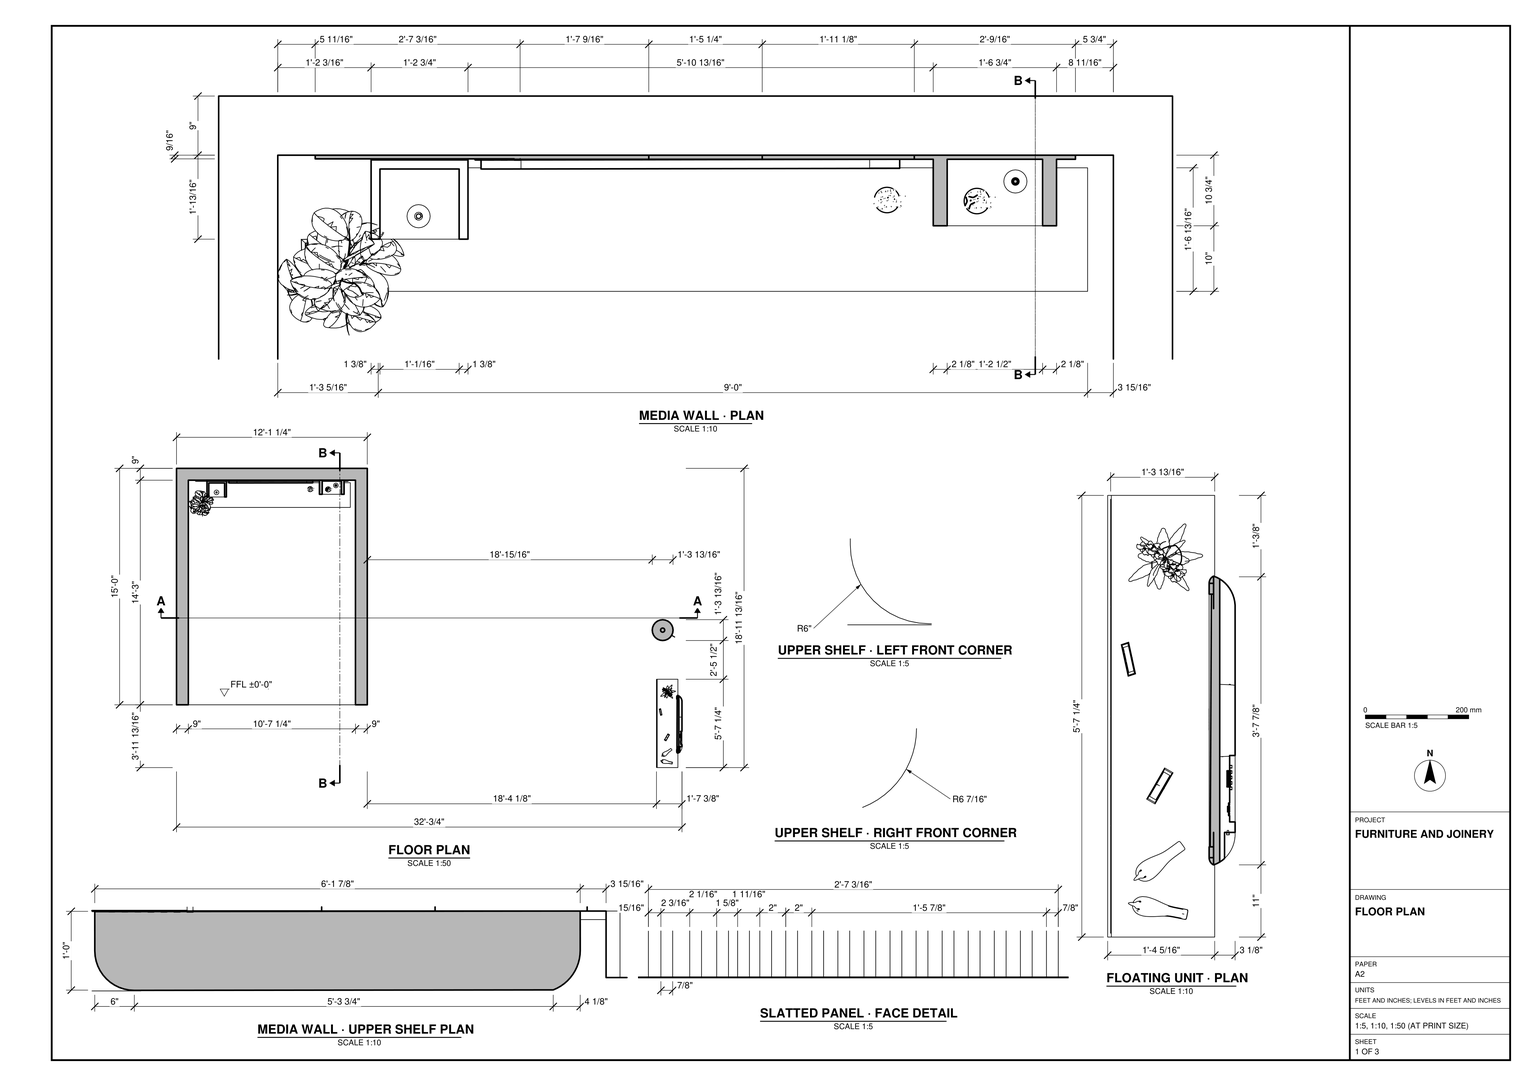
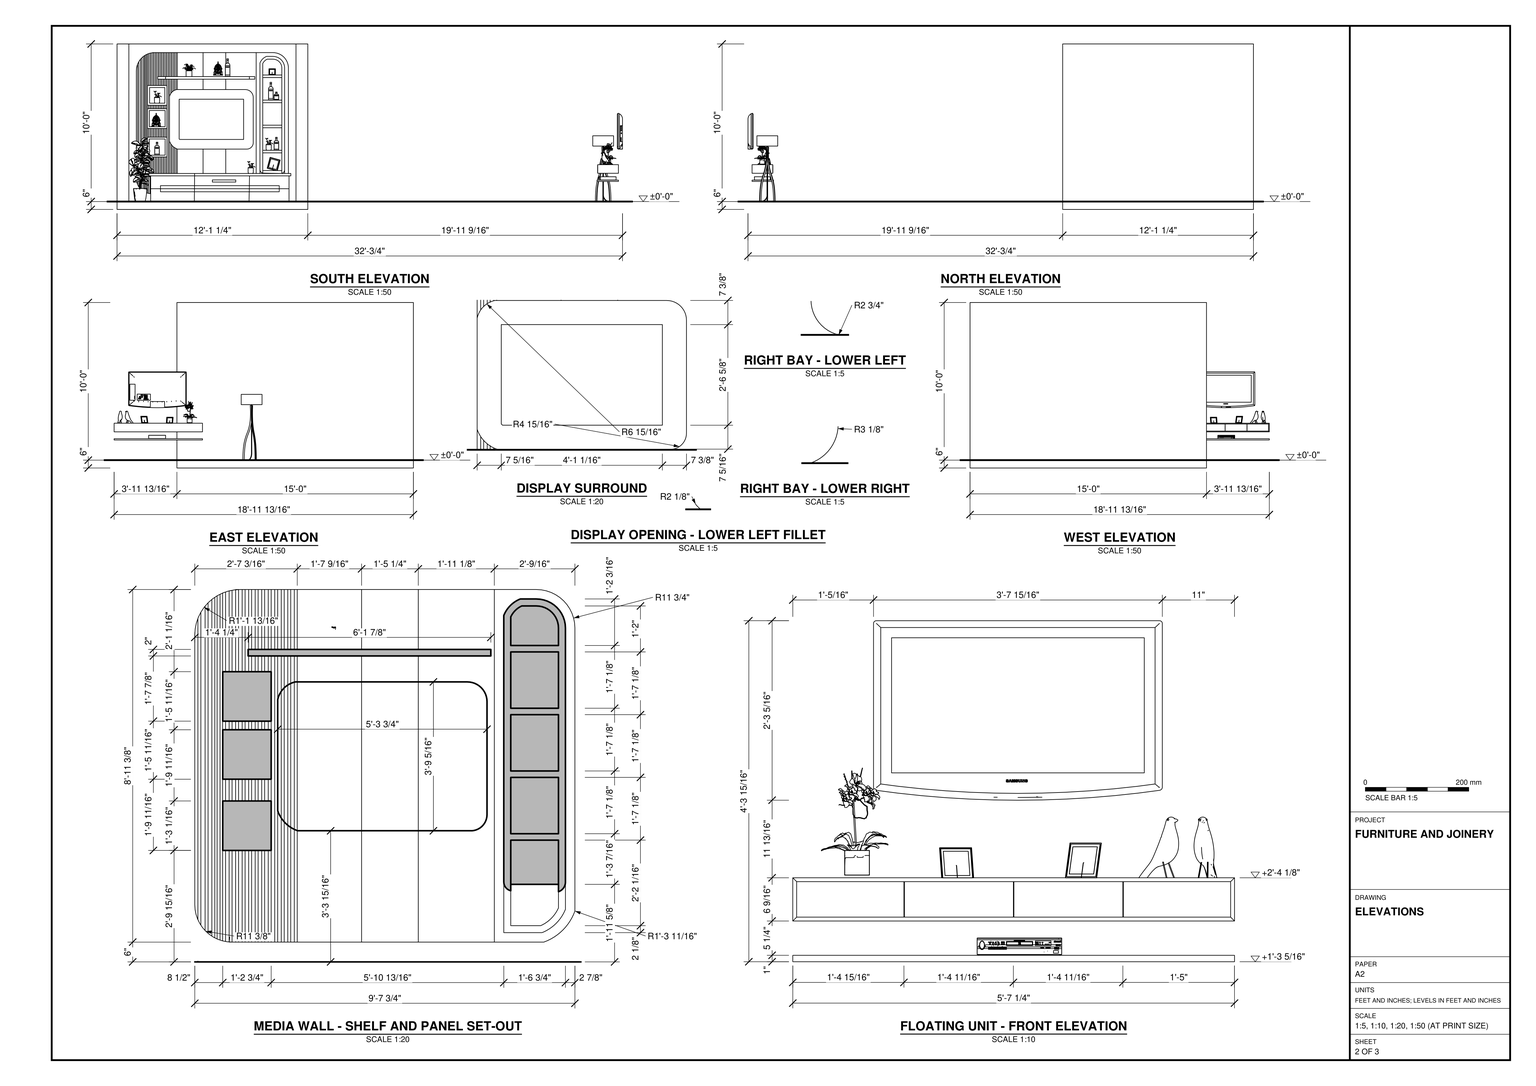
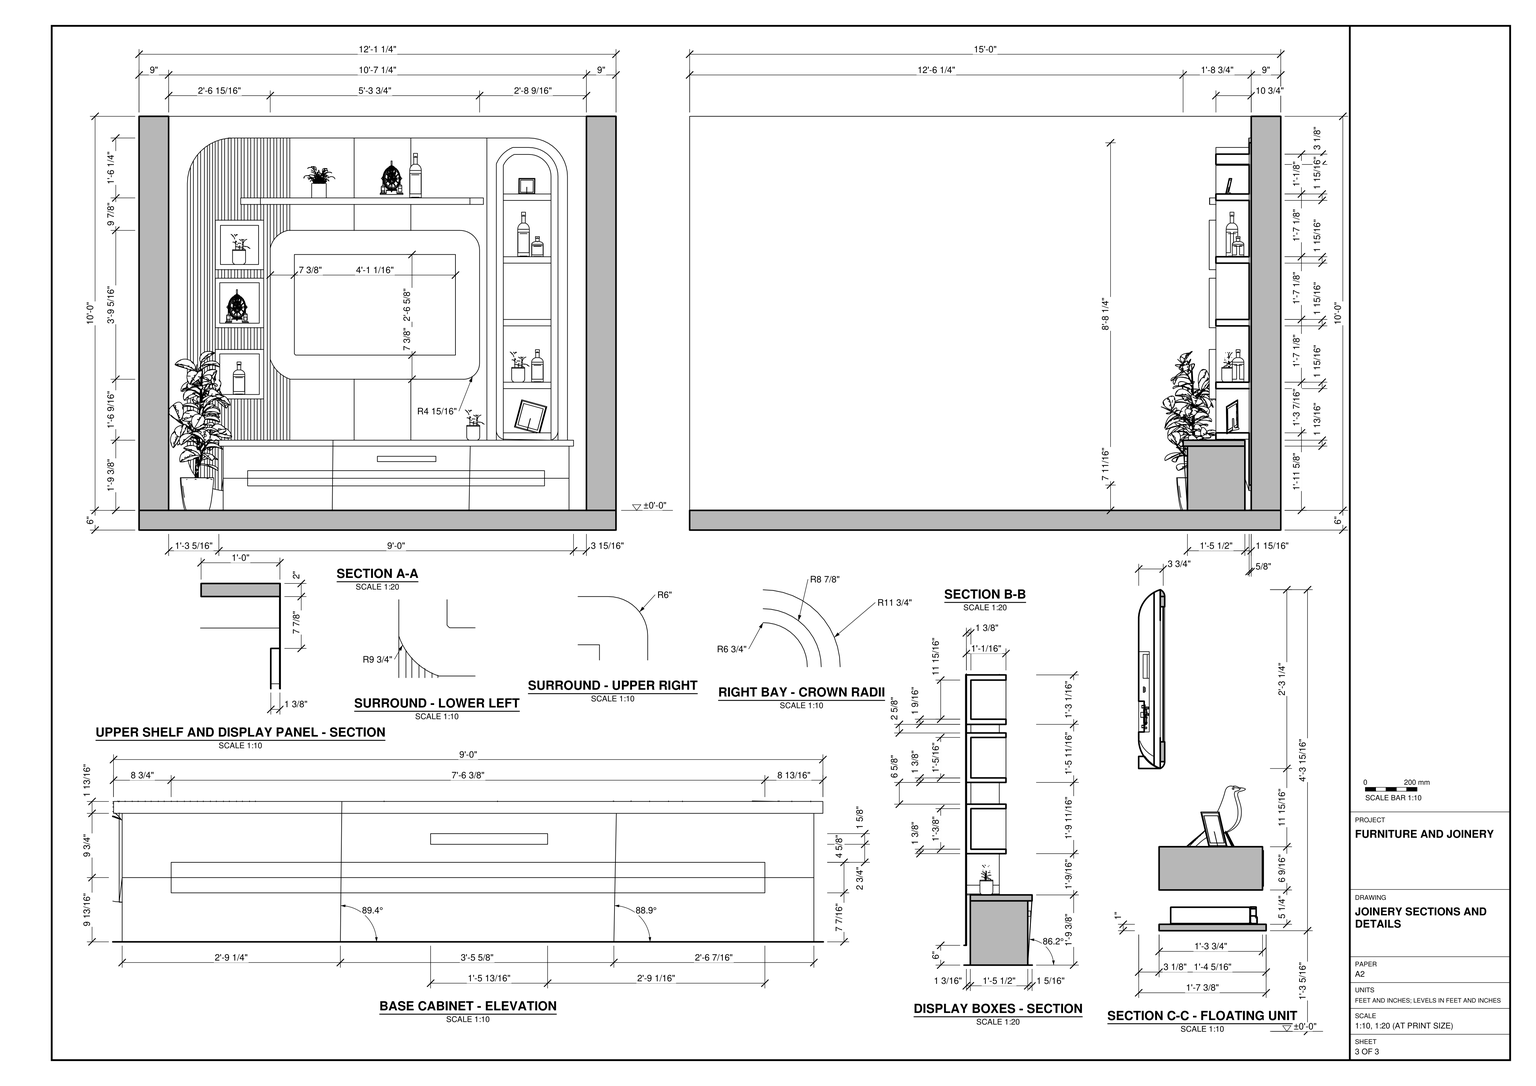
Use task_files/diagram_01.pdf to build the media wall, its enclosure and the separate floating display unit in SketchUp. Work in feet and inches. The complete layout measures 32'-3/4" along x, 18'-11 13/16" along y and 10'-6" in height. Set the single finished floor level at ±0'-0". Model the 6" floor slab and the 9" back and side walls, leaving the front open as shown in plan.

Build the media wall against the back wall. Use the section facing the joinery to align the divided base cabinet, slatted panel, three open display boxes, central display surround and tall right-hand shelving bay. Follow the details for the rounded corners of the surround, the projecting upper shelf and the nested curves at the crown of the shelving bay.

Use the floor plan to position the separate floating unit outside the enclosure, with its length perpendicular to the base cabinet. Include its divided console, lower shelf and display above. Decor and loose items, including plants, clocks, lamps and objects on the shelves, may be any suitable library components placed as shown. Keep the walls, slab and each furniture or joinery piece in separate groups or components, and use components for repeated parts. Save one SketchUp model as output_files/media_wall_and_separate_floating_display_unit.skp.

# SketchUp Ruby script. Lengths in inches.
U = 1.inch
M = Sketchup.active_model
def pt(a) = Geom::Point3d.new(a.map { |v| v * U })
def face(e, loops, mat)
  f = e.add_face(loops[0].map { |a| pt(a) })
  loops[1..].each { |l| e.add_face(l.map { |a| pt(a) }).erase! }
  f.material = f.back_material = mat if mat
  f
end
# faces: each face lists its corners as indices into pts; further lists are holes
def faces(e, pts, list, mat = nil) = list.each { |f| face(e, (f[0].is_a?(Array) ? f : [f]).map { |l| l.map { |i| pts[i] } }, mat) }
# xy, xz, yz: faces in a plane at the given z, y or x. An outline is a flat list of corners, or four numbers for a rectangle; further outlines are holes
def ring(l) = l.size == 4 ? [[l[0], l[1]], [l[2], l[1]], [l[2], l[3]], [l[0], l[3]]] : l.each_slice(2).to_a
def flat(e, list, mat, &to3) = list.each { |f| face(e, (f[0].is_a?(Array) ? f : [f]).map { |l| ring(l).map { |u, v| to3.(u, v) } }, mat) }
def xy(e, z, list, mat = nil) = flat(e, list, mat) { |x, y| [x, y, z] }
def xz(e, y, list, mat = nil) = flat(e, list, mat) { |x, z| [x, y, z] }
def yz(e, x, list, mat = nil) = flat(e, list, mat) { |y, z| [x, y, z] }
def lines(e, pts, list) = list.each { |a, b| e.add_line(pt(pts[a]), pt(pts[b])) }
# prism: a flat outline (further loops are holes) pulled along v
def prism(e, loops, v, mat = nil)
  f = face(e, loops, mat); d = Geom::Vector3d.new(v.map { |x| x * U })
  f.pushpull(f.normal.samedirection?(d) ? d.length : -d.length)
end
def box(e, o, s, mat = nil) = prism(e, [[o, [o[0] + s[0], o[1], o[2]], [o[0] + s[0], o[1] + s[1], o[2]], [o[0], o[1] + s[1], o[2]]]], [0, 0, s[2]], mat)
def at(x, y, z, deg = 0) = Geom::Transformation.translation(pt([x, y, z])) * Geom::Transformation.rotation(ORIGIN, Z_AXIS, deg.degrees)
def axes(o, x, y, z) = Geom::Transformation.new([*x, 0, *y, 0, *z, 0, *pt(o).to_a, 1])
def part(name) = M.definitions.add(name)
# library, detail: a bought-in or finely detailed component or shape, given as its bounding box
def library(name, o, s) = part(name).tap { |d| box(d.entities, o, s) }
def detail(e, o, s) = box(e.add_group.entities, o, s)
def put(e, d, t, mat = nil) = e.add_instance(d, t).tap { |i| i.material = mat if mat }
def group(e, t, mat = nil) = e.add_group.tap { |g| g.transformation = t; g.material = mat if mat }.entities
root = M.entities
M.materials.add("Frame_Pic").color = [0, 0, 0]
M.materials.add("Glossy_White").color = [188, 188, 188]
M.materials.add("Pic_Bed").color = [214, 209, 200]
M.materials.add("White Wall").color = [242, 239, 237]
M.materials.add("White_Fur").color = [226, 226, 226]
M.materials.add("Wood_Fur").color = [191, 176, 157]
M.materials.add("[Blinds Vertical Pattern]").color = [212, 212, 214]
M.materials.add("[Color M00]").color = [255, 255, 255]
M.materials.add("[Color M09]").color = [0, 0, 0]
M.materials.add("[Color_000]1").color = [255, 255, 126]
M.materials.add("[Color_000]2").color = [135, 140, 128]
M.materials.add("[Color_008]1").color = [28, 28, 28]
M.materials.add("[Color_008]2").color = [29, 29, 29]
M.materials.add("[Wood Bamboo]").color = [177, 105, 43]
M.materials.add("kinh1").color = [126, 126, 126]
M.materials["kinh1"].alpha = 0
M.materials.add("model").color = [217, 78, 64]
M.materials.add("product_RG_W___dLorraine_80x80_Kepingan2").color = [228, 228, 223]
c1 = library("Small Plant for Nightstand",[-0.92,-1.74,0],[6.62,5.06,9.81])
c2 = library("PLANT SMALL",[-1.72,-1.35,0],[13.55,13.62,9.59])
c3 = library("SmallMag",[0,-0.13,0],[5.12,2.39,5.75])
c4 = library("Vodka",[0,0,0],[3.53,3.53,13.57])
c5 = library("Group_2",[-1.28,-0.39,0],[21.22,20.51,48.44])
c6 = library("model",[-3.64,-1.86,0],[7.28,3.72,11.8125])
c7 = library("Estante p/ Sala de TV - designed by Tiago Crisostomo",[-3.75,0,10.71],[23.44,133.86,62.71])
c8 = library("Potted orchid",[-4.6,-2.59,0],[19.81,21.87,25.9])
c9 = part("Group\#70")
xy(c9.entities,0,[[0,0,16.59,0.1]],"Glossy_White")
xy(c9.entities,5.4,[[0,0,16.59,0.1]],"Glossy_White")
xz(c9.entities,0,[[0,0,16.59,5.4]])
xz(c9.entities,0.1,[[0,0,16.59,5.4]],"Glossy_White")
yz(c9.entities,0,[[0,0,0.1,5.4]],"Glossy_White")
yz(c9.entities,16.59,[[0,0,0.1,5.4]],"Glossy_White")
c10 = part("Group\#83")
xy(c10.entities,0,[[0.26,0,16.59,0.1]],"Glossy_White")
xy(c10.entities,5.4,[[0.26,0,16.59,0.1]],"Glossy_White")
xz(c10.entities,0,[[0.26,0,16.59,5.4]])
xz(c10.entities,0.1,[[0.26,0,16.59,5.4]],"Glossy_White")
yz(c10.entities,0.26,[[0,0,0.1,5.4]],"Glossy_White")
yz(c10.entities,16.59,[[0,0,0.1,5.4]],"Glossy_White")
c11 = library("Group\#74",[-0.65,-0.12,0],[14.95,9.57,9.38])
c12 = part("Picture frame stand")
prism(c12.entities,[[[0,6.65,1.14],[0,6.68,0.91],[0,6.65,0.68],[0,6.5625,0.47],[0,6.43,0.28],[0,6.25,0.14],[0,6.04,0.04],[0,5.82,0],[0,0,0],[0,2.74,10.21],[0,2.79,10.35],[0,2.87,10.47],[0,2.98,10.57],[0,3.1,10.65],[0,3.24,10.7],[0,3.39,10.71],[0,3.53,10.7],[0,3.67,10.65],[0,3.8,10.57],[0,3.9,10.47],[0,3.99,10.35],[0,4.04,10.21],[0,2.39,3.68],[0,2.35,3.44],[0,2.35,3.2],[0,2.39,2.96],[0,2.47,2.73],[0,2.58,2.51],[0,2.72,2.32],[0,2.9,2.15],[0,3.1,2.01],[0,3.32,1.91],[0,3.55,1.84],[0,3.8,1.81],[0,4.04,1.82],[0,5.82,1.82],[0,6.04,1.78],[0,6.25,1.68],[0,6.43,1.54],[0,6.5625,1.35]]],[0.2,0,0],"Frame_Pic")
c13 = part("Standing picture frame")
yz(c13.entities,0,[[0.38,0,0,0.1,6.52,24.44,6.9,24.34]],"Frame_Pic")
yz(c13.entities,0.79,[[0.58,0.76,6.7,23.58,6.51,23.63,0.39,0.8125],[0.39,0.8125,6.51,23.63,6.32,23.68,0.2,0.86]])
yz(c13.entities,2.76,[[0.9,2.71,0.71,2.76,5.81,21.78,6,21.73]],"[Color_008]1")
yz(c13.entities,22.44,[[0.9,2.71,6,21.73,5.81,21.78,0.71,2.76]],"[Color_008]1")
yz(c13.entities,24.41,[[0.58,0.76,0.39,0.8125,6.51,23.63,6.7,23.58]])
yz(c13.entities,24.41,[[0.39,0.8125,0.2,0.86,6.32,23.68,6.51,23.63]],"[Color_008]1")
yz(c13.entities,25.2,[[0.38,0,6.9,24.34,6.52,24.44,0,0.1]],"Frame_Pic")
p = [[0,0.38,0],[25.2,0.38,0],[25.2,0,0.1],[0,0,0.1],[0,6.9,24.34],[25.2,6.9,24.34],
  [24.41,6.7,23.58],[0.79,6.7,23.58],[0.79,0.58,0.76],[24.41,0.58,0.76],[0,6.52,24.44],[25.2,6.52,24.44],
  [0.79,6.32,23.68],[24.41,6.32,23.68],[24.41,0.2,0.86],[0.79,0.2,0.86],[24.41,0.39,0.8125],[0.79,0.39,0.8125],
  [24.41,6.51,23.63],[0.79,6.51,23.63],[22.44,6,21.73],[22.44,0.9,2.71],[2.76,0.9,2.71],[2.76,6,21.73],
  [2.76,0.71,2.76],[22.44,0.71,2.76],[22.44,5.81,21.78],[2.76,5.81,21.78]]
faces(c13.entities,p,[[0,1,2,3],[[0,4,5,1],[6,7,8,9]],[14,16,17,15],[24,22,21,25],[26,20,23,27]],"[Color_008]1")
faces(c13.entities,p,[[[10,3,2,11],[12,13,14,15]],[5,4,10,11]],"Frame_Pic")
faces(c13.entities,p,[[[16,18,19,17],[20,21,22,23]],[7,6,9,8]],"[Color_000]2")
faces(c13.entities,p,[[9,8,17,16],[21,20,23,22],[12,19,18,13],[7,6,18,19]])
faces(c13.entities,p,[[24,25,26,27]],"Pic_Bed")
put(c13.entities,c12,at(12.6,0.38,0))
c14 = part("Picture frame stand \#1")
prism(c14.entities,[[[0.2,0,0],[0.2,5.82,0],[0.2,6.04,0.04],[0.2,6.25,0.14],[0.2,6.43,0.28],[0.2,6.5625,0.47],[0.2,6.65,0.68],[0.2,6.68,0.91],[0.2,6.65,1.14],[0.2,6.5625,1.35],[0.2,6.43,1.54],[0.2,6.25,1.68],[0.2,6.04,1.78],[0.2,5.82,1.82],[0.2,4.04,1.82],[0.2,3.8,1.81],[0.2,3.55,1.84],[0.2,3.32,1.91],[0.2,3.1,2.01],[0.2,2.9,2.15],[0.2,2.72,2.32],[0.2,2.58,2.51],[0.2,2.47,2.73],[0.2,2.39,2.96],[0.2,2.35,3.2],[0.2,2.35,3.44],[0.2,2.39,3.68],[0.2,4.04,10.21],[0.2,3.99,10.35],[0.2,3.9,10.47],[0.2,3.8,10.57],[0.2,3.67,10.65],[0.2,3.53,10.7],[0.2,3.39,10.71],[0.2,3.24,10.7],[0.2,3.1,10.65],[0.2,2.98,10.57],[0.2,2.87,10.47],[0.2,2.79,10.35],[0.2,2.74,10.21]]],[-0.2,0,0],"[Color_008]1")
c15 = part("Standing picture frame \#1")
yz(c15.entities,0,[[0.38,0,0,0.1,6.52,24.44,6.9,24.34]],"[Color_008]2")
yz(c15.entities,0.79,[[0.58,0.76,6.7,23.58,6.51,23.63,0.39,0.8125],[0.39,0.8125,6.51,23.63,6.32,23.68,0.2,0.86]])
yz(c15.entities,2.76,[[0.9,2.71,0.71,2.76,5.81,21.78,6,21.73]],"[Color_008]2")
yz(c15.entities,22.44,[[0.9,2.71,6,21.73,5.81,21.78,0.71,2.76]],"[Color_008]2")
yz(c15.entities,24.41,[[0.58,0.76,0.39,0.8125,6.51,23.63,6.7,23.58]])
yz(c15.entities,24.41,[[0.39,0.8125,0.2,0.86,6.32,23.68,6.51,23.63]],"[Color_008]2")
yz(c15.entities,25.2,[[0.38,0,6.9,24.34,6.52,24.44,0,0.1]],"[Color_008]2")
p = [[0,0.38,0],[25.2,0.38,0],[25.2,0,0.1],[0,0,0.1],[0,6.9,24.34],[25.2,6.9,24.34],
  [24.41,6.7,23.58],[0.79,6.7,23.58],[0.79,0.58,0.76],[24.41,0.58,0.76],[0,6.52,24.44],[0.05,-0.6,0.22],
  [0.05,5.92,24.55],[25.25,-0.6,0.22],[25.2,6.52,24.44],[25.25,5.92,24.55],[0.84,5.72,23.79],[24.46,5.72,23.79],
  [24.46,-0.4,0.98],[0.84,-0.4,0.98],[24.41,0.2,0.86],[24.41,0.39,0.8125],[0.79,0.39,0.8125],[0.79,0.2,0.86],
  [24.41,6.51,23.63],[0.79,6.51,23.63],[22.44,6,21.73],[22.44,0.9,2.71],[2.76,0.9,2.71],[2.76,6,21.73],
  [0.79,6.32,23.68],[24.41,6.32,23.68],[2.76,0.71,2.76],[22.44,0.71,2.76],[22.44,5.81,21.78],[2.76,5.81,21.78]]
faces(c15.entities,p,[[0,1,2,3],[[0,4,5,1],[6,7,8,9]],[10,3,11,12],[3,2,13,11],[2,14,15,13],[[12,11,13,15],[16,17,18,19]],[20,21,22,23],[23,30,16,19],
  [20,23,19,18],[31,20,18,17],[32,28,27,33],[34,26,29,35],[30,31,17,16],[5,4,10,14],[14,10,12,15]],"[Color_008]2")
faces(c15.entities,p,[[[21,24,25,22],[26,27,28,29]],[7,6,9,8]],"[Color_000]1")
faces(c15.entities,p,[[9,8,22,21],[27,26,29,28],[32,33,34,35],[30,25,24,31],[7,6,24,25]])
put(c15.entities,c14,at(12.6,0.38,0))
c16 = part("Standing picture frame \#2")
yz(c16.entities,0,[[0.38,0,0,0.1,6.52,24.44,6.9,24.34]],"[Color_008]2")
yz(c16.entities,0.79,[[0.58,0.76,6.7,23.58,6.51,23.63,0.39,0.8125],[0.39,0.8125,6.51,23.63,6.32,23.68,0.2,0.86]])
yz(c16.entities,2.76,[[0.9,2.71,0.71,2.76,5.81,21.78,6,21.73]],"[Color_008]2")
yz(c16.entities,22.44,[[0.9,2.71,6,21.73,5.81,21.78,0.71,2.76]],"[Color_008]2")
yz(c16.entities,24.41,[[0.58,0.76,0.39,0.8125,6.51,23.63,6.7,23.58]])
yz(c16.entities,24.41,[[0.39,0.8125,0.2,0.86,6.32,23.68,6.51,23.63]],"[Color_008]2")
yz(c16.entities,25.2,[[0.38,0,6.9,24.34,6.52,24.44,0,0.1]],"[Color_008]2")
p = [[0,0.38,0],[25.2,0.38,0],[25.2,0,0.1],[0,0,0.1],[0,6.9,24.34],[25.2,6.9,24.34],
  [24.41,6.7,23.58],[0.79,6.7,23.58],[0.79,0.58,0.76],[24.41,0.58,0.76],[0,6.52,24.44],[0.05,-0.6,0.22],
  [0.05,5.92,24.55],[25.25,-0.6,0.22],[25.2,6.52,24.44],[25.25,5.92,24.55],[0.84,5.72,23.79],[24.46,5.72,23.79],
  [24.46,-0.4,0.98],[0.84,-0.4,0.98],[24.41,0.2,0.86],[24.41,0.39,0.8125],[0.79,0.39,0.8125],[0.79,0.2,0.86],
  [24.41,6.51,23.63],[0.79,6.51,23.63],[22.44,6,21.73],[22.44,0.9,2.71],[2.76,0.9,2.71],[2.76,6,21.73],
  [0.79,6.32,23.68],[24.41,6.32,23.68],[2.76,0.71,2.76],[22.44,0.71,2.76],[22.44,5.81,21.78],[2.76,5.81,21.78]]
faces(c16.entities,p,[[0,1,2,3],[[0,4,5,1],[6,7,8,9]],[10,3,11,12],[3,2,13,11],[2,14,15,13],[[12,11,13,15],[16,17,18,19]],[20,21,22,23],[23,30,16,19],
  [20,23,19,18],[31,20,18,17],[32,28,27,33],[34,26,29,35],[30,31,17,16],[5,4,10,14],[14,10,12,15]],"[Color_008]2")
faces(c16.entities,p,[[9,8,22,21],[27,26,29,28],[32,33,34,35],[30,25,24,31],[7,6,24,25]])
faces(c16.entities,p,[[[21,24,25,22],[26,27,28,29]],[7,6,9,8]],"[Color_000]1")
put(c16.entities,c14,at(12.6,0.38,0))
c17 = library("Groupe\#5",[0,0,0],[91.34,77.95,241.79])
c18 = part("1+(1)")
g1 = group(c18.entities,at(22.63,0,15.32,90))
put(g1,c7,axes([0,3.11,-8.87],[0,0.828,0],[0.50243,0,0],[0,0,0.828]),"White Wall")
put(g1,c8,axes([53.95,5.4,13.18],[0.64,0,0],[0,0.64,0],[0,0,0.64]))
g2 = group(g1,at(0,3.11,6.2))
xy(g2,0,[[0,0,67.25,15.75]],"Wood_Fur")
xy(g2,6.58,[[0,0,67.25,15.75]],"White_Fur")
xz(g2,0,[[0,0,67.25,6.58]],"Glossy_White")
xz(g2,15.75,[[0,0,0,6.58,0.59,5.99,0.59,0.59],[0,0,0.59,0.59,0.59,5.99,0,6.58,67.25,6.58,66.66,5.99,66.66,0.59,67.25,0],[67.25,0,66.66,0.59,66.66,5.99,67.25,6.58]],"Wood_Fur")
yz(g2,0,[[0,0,15.75,6.58]],"Wood_Fur")
yz(g2,67.25,[[0,0,15.75,6.58]],"Glossy_White")
put(g2,c9,at(33.67,15.75,0.59))
put(g2,c9,at(17,15.75,0.59))
put(g2,c10,at(0.33,15.75,0.59))
put(g2,c10,at(50.08,15.75,0.59))
put(g1,c11,at(14.57,16.25,12.65,180))
g3 = group(g1,at(21.54,4.37,12.79,15))
put(g3,c13,axes([255.49,207.07,-2.77],[-0.20896,-0.25753,-0.08299],[0.25289,-0.22317,0.05582],[-0.09622,-0.02727,0.32691]))
put(g3,c13,axes([5.73,5.06,-0.02],[-0.15397,0.15397,0],[-0.15397,-0.15397,0],[0,0,0.21775]))
g4 = group(g1,at(50.59,15.13,12.6))
g5 = group(g4,at(163.33,253.62,68.43))
put(g5,c15,axes([-2.84,-4.49,0],[0.0285,0.19491,0],[0.16454,-0.00675,0],[0,0,0.19429]))
g6 = group(g5,at(-0.1875,-0.07,0.125),"kinh1")
prism(g6,[[[-1.64,-4.36,4.54],[-2.67,-4.32,0],[-1.98,0.4,0],[-0.95,0.36,4.54]]],[-0.01,0,0])
g7 = group(g4,at(-5.67,0,0))
put(g7,c16,axes([-5.21,1.08,0],[0.19248,0.04191,0],[0.05157,-0.15639,0],[0,0,0.19429]))
g8 = group(g7,at(-0.13,0.15,0.125),"kinh1")
prism(g8,[[[-4.66,0,4.54],[-4.98,0.98,0],[-0.32,1.99,0],[0,1.01,4.54]]],[0,0.01,0])
put(c18.entities,c17,axes([21.1,106.21,0],[-0.176,0.10161,0],[-0.10161,-0.176,0],[0,0,0.2071]))
xy(root,6.026,[[45,218.054,45.899,218.179],[43.015,218.06,43.914,218.185],[41.031,218.067,41.929,218.192],[39.046,218.073,39.945,218.198],[37.061,218.079,37.96,218.204],
  [35.077,218.085,35.975,218.21],[33.092,218.092,33.991,218.217],[31.107,218.098,32.006,218.223],[29.123,218.104,30.021,218.229],[27.138,218.11,28.036,218.235],
  [25.153,218.117,26.052,218.242],[45,218.179,45.899,218.804],[45.899,218.179,65.488,218.242],[65.488,218.179,82.758,218.804],[82.758,218.179,105.912,218.804],
  [105.912,218.179,120.978,218.804],[26.052,218.242,45,218.804],[45.899,218.242,65.488,218.804]])
xy(root,23.613,[[110.916,208.054,125.443,218.179]])
xy(root,33.941,[[23.21,206.017,37.96,218.079]])
xy(root,35.289,[[24.557,206.017,36.612,216.701]])
xy(root,37.08,[[110.916,208.054,125.443,218.179]])
xy(root,39.034,[[110.916,208.054,125.443,218.179]])
xy(root,47.656,[[24.557,206.017,36.612,216.701]])
xy(root,49.004,[[23.21,206.017,37.96,218.079]])
xy(root,55.632,[[23.21,206.017,37.96,218.079]])
xy(root,56.184,[[110.916,208.054,125.443,218.179]])
xy(root,56.997,[[24.574,206.017,36.596,216.701]])
xy(root,58.138,[[110.916,208.054,125.443,218.179]])
xy(root,69.331,[[24.574,206.017,36.596,216.701]])
xy(root,70.695,[[23.21,206.017,37.96,218.079]])
xy(root,73.305,[[23.21,206.017,37.96,218.079]])
xy(root,74.879,[[24.784,206.017,36.386,216.701]])
xy(root,75.288,[[110.916,208.054,125.443,218.179]])
xy(root,77.242,[[110.916,208.054,125.443,218.179]])
xy(root,86.794,[[24.784,206.017,36.386,216.701]])
xy(root,88.368,[[23.21,206.017,37.96,218.079]])
xy(root,94.392,[[110.916,208.054,125.443,218.179]])
xy(root,96.347,[[110.916,208.054,125.443,218.179]])
xy(root,108.396,[[114.25,208.054,118.709,218.179]])
xy(root,110.519,[[113.802,208.054,118.709,218.179]])
xy(root,113.401,[[45,218.054,45.899,218.179],[43.015,218.06,43.914,218.185],[41.031,218.067,41.929,218.192],[39.046,218.073,39.945,218.198],[37.061,218.079,37.96,218.204],
  [35.077,218.085,35.975,218.21],[33.092,218.092,33.991,218.217],[31.107,218.098,32.006,218.223],[29.123,218.104,30.021,218.229],[27.138,218.11,28.036,218.235],
  [45,218.179,45.899,218.179,45.899,218.242,65.488,218.242,65.488,218.804,28.506,218.804,28.506,218.242,45,218.242],[45.899,218.179,65.488,218.242],[65.488,218.179,82.758,218.804],[82.758,218.179,105.912,218.804],[105.912,218.179,118.709,218.804]])
xz(root,206.017,[[[23.21,33.941,37.96,49.004],[24.557,35.289,36.612,47.656]],[[23.21,55.632,37.96,70.695],[24.574,56.997,36.596,69.331]]])
xz(root,206.017,[[[23.21,73.305,37.96,88.368],[24.784,74.879,36.386,86.794]]],"[Color M00]")
xz(root,208.054,[[125.443,21.375,125.744,21.494,126.031,21.643,126.301,21.821,126.551,22.026,126.778,22.256,126.98,22.509,127.155,22.781,127.301,23.07,127.416,23.372,127.499,23.685,127.549,24.004,127.566,24.327,127.566,101.662,127.49,102.819,127.264,103.955,126.892,105.052,126.38,106.091,125.736,107.054,124.972,107.925,124.101,108.689,123.138,109.333,122.099,109.845,121.002,110.218,119.865,110.444,118.709,110.519,113.802,110.519,113.247,110.274,112.71,109.993,112.193,109.676,111.698,109.325,111.229,108.941,110.786,108.527,110.371,108.084,109.988,107.614,109.637,107.119,109.32,106.602,109.038,106.065,108.793,105.51,108.793,24.342,108.81,24.036,108.861,23.734,108.946,23.44,109.063,23.156,109.212,22.888,109.389,22.638,109.593,22.409,109.821,22.205,110.071,22.027,110.339,21.879,110.622,21.761,110.916,21.676,110.916,105.0625,110.952,105.143,111.167,105.553,111.409,105.949,111.678,106.327,111.971,106.686,112.288,107.025,112.626,107.341,112.986,107.635,113.364,107.903,113.759,108.146,114.17,108.361,114.25,108.396,118.709,108.396,119.588,108.339,120.452,108.167,121.286,107.884,122.076,107.494,122.808,107.005,123.471,106.424,124.051,105.762,124.541,105.029,124.93,104.239,125.213,103.405,125.385,102.541,125.443,101.662],[125.443,21.375,125.443,23.613,110.916,23.613,110.916,21.676],[110.916,37.08,125.443,39.034],[110.916,56.184,125.443,58.138],[110.916,75.288,125.443,77.242],
  [110.916,94.392,125.443,96.347]],"[Color M09]")
xz(root,216.701,[[24.557,35.289,36.612,47.656],[24.574,56.997,36.596,69.331],[24.784,74.879,36.386,86.794]])
xz(root,218.054,[[45,6.026,45.899,113.401]],"[Wood Bamboo]")
xz(root,218.06,[[43.015,6.026,43.914,113.401]])
xz(root,218.067,[[41.031,6.026,41.929,113.401]],"[Blinds Vertical Pattern]")
xz(root,218.073,[[39.046,6.026,39.945,113.401]])
xz(root,218.079,[[37.061,6.026,37.96,33.941],[23.21,33.941,37.061,49.004],[37.061,33.941,37.96,49.004],[37.061,49.004,37.96,55.632],[23.21,55.632,37.061,70.695],
  [37.061,55.632,37.96,70.695],[37.061,70.695,37.96,73.305],[23.21,73.305,37.061,88.368],[37.061,73.305,37.96,88.368],[37.061,88.368,37.96,113.401]])
xz(root,218.085,[[35.077,6.026,35.975,113.401]])
xz(root,218.092,[[33.092,6.026,33.991,113.401]])
xz(root,218.098,[[31.107,6.026,32.006,113.401]])
xz(root,218.104,[[29.123,6.026,30.021,113.401]])
xz(root,218.11,[[27.138,6.026,28.036,113.401]])
xz(root,218.117,[[25.153,6.026,26.052,6.026,26.052,113.153,25.153,112.989]])
xz(root,218.179,[[45,6.026,45.899,113.401],[[105.912,6.026,120.978,6.026,122.048,6.455,123.083,6.961,124.079,7.542,125.029,8.195,125.929,8.915,126.773,9.7,127.558,10.544,128.279,11.444,128.931,12.394,129.512,13.39,130.019,14.425,130.448,15.495,130.448,101.662,130.347,103.195,130.048,104.701,129.554,106.155,128.875,107.532,128.022,108.808,127.009,109.963,125.855,110.975,124.578,111.828,123.201,112.507,121.747,113.001,120.241,113.3,118.709,113.401,105.912,113.401],[108.793,8.907,108.793,105.51,109.038,106.065,109.32,106.602,109.637,107.119,109.988,107.614,110.371,108.084,110.786,108.527,111.229,108.941,111.698,109.325,112.193,109.676,112.71,109.993,113.247,110.274,113.802,110.519,118.709,110.519,119.865,110.444,121.002,110.218,122.099,109.845,123.138,109.333,124.101,108.689,124.972,107.925,125.736,107.054,126.38,106.091,126.892,105.052,127.264,103.955,127.49,102.819,127.566,101.662,127.566,16.051,127.384,15.596,126.97,14.751,126.496,13.938,125.963,13.163,125.375,12.428,124.735,11.739,124.045,11.098,123.311,10.51,122.535,9.977,121.723,9.503,120.877,9.09,120.422,8.907]],[108.793,8.907,120.422,8.907,120.877,9.09,121.723,9.503,122.535,9.977,123.311,10.51,124.045,11.098,124.735,11.739,125.375,12.428,125.963,13.163,126.496,13.938,126.97,14.751,127.384,15.596,127.566,16.051,127.566,24.327,127.549,24.004,127.499,23.685,127.416,23.372,127.301,23.07,127.155,22.781,126.98,22.509,126.778,22.256,126.551,22.026,126.301,21.821,126.031,21.643,125.744,21.494,125.443,21.375,125.443,16.461,125.442,16.459,125.097,15.754,124.701,15.076,124.257,14.429,123.767,13.816,123.232,13.241,122.657,12.707,122.045,12.216,121.398,11.772,120.72,11.376,120.015,11.032,120.012,11.031,110.916,11.031,110.916,21.676,110.622,21.761,110.339,21.879,110.071,22.027,109.821,22.205,109.593,22.409,109.389,22.638,109.212,22.888,109.063,23.156,108.946,23.44,108.861,23.734,108.81,24.036,108.793,24.342],[110.916,11.031,120.012,11.031,120.015,11.032,120.72,11.376,121.398,11.772,122.045,12.216,122.657,12.707,123.232,13.241,123.767,13.816,124.257,14.429,124.701,15.076,125.097,15.754,125.442,16.459,125.443,16.461,125.443,23.613,110.916,23.613],[110.916,39.034,125.443,56.184],
  [110.916,58.138,125.443,75.288],[110.916,77.242,125.443,94.392],[110.916,96.347,125.443,96.347,125.443,101.662,125.385,102.541,125.213,103.405,124.93,104.239,124.541,105.029,124.051,105.762,123.471,106.424,122.808,107.005,122.076,107.494,121.286,107.884,120.452,108.167,119.588,108.339,118.709,108.396,114.25,108.396,114.17,108.361,113.759,108.146,113.364,107.903,112.986,107.635,112.626,107.341,112.288,107.025,111.971,106.686,111.678,106.327,111.409,105.949,111.167,105.553,110.952,105.143,110.916,105.0625]])
xz(root,218.179,[[45.899,6.026,65.488,113.401],[65.488,6.026,82.758,113.401],[82.758,6.026,105.912,113.401]],"product_RG_W___dLorraine_80x80_Kepingan2")
xz(root,218.242,[[26.052,6.026,25.153,6.085,25.153,112.974,26.052,113.153],[24.077,6.221,24.077,112.64,23.222,112.35,23.178,112.328,23.178,6.4],[22.39,6.658,22.39,111.94,21.602,111.551,21.491,111.477,21.491,6.996,21.707,6.89],[20.796,7.339,20.796,111.012,20.1,110.547,19.897,110.37,19.897,7.866,20.375,7.547],[18.742,8.721,18.742,109.356,17.843,108.332,17.843,9.556,18.023,9.351],
  [16.548,11.211,16.548,106.497,15.749,104.877,15.649,104.583,15.649,12.858,16.219,11.703]])
xz(root,218.242,[[26.052,6.026,45,6.026,45,113.401,28.506,113.401,26.703,113.283,26.052,113.153],[25.153,6.085,25.153,112.974,24.932,112.93,24.077,112.64,24.077,6.221,24.57,6.123],[23.178,6.4,23.178,112.328,22.39,111.94,22.39,6.658,23.113,6.413],[21.491,6.996,21.491,111.477,20.796,111.012,20.796,7.339],[19.897,7.866,19.897,110.37,18.742,109.356,18.742,8.721,19.14,8.372],
  [17.843,9.556,17.843,108.332,17.551,107.999,16.548,106.497,16.548,11.211,17.044,10.468],[15.649,12.858,15.649,104.583,15.168,103.166,14.816,101.395,14.698,99.593,14.698,17.38,14.795,15.898,15.084,14.441,15.562,13.035]],"[Wood Bamboo]")
xz(root,218.804,[[26.052,6.026,24.57,6.123,23.113,6.413,21.707,6.89,20.375,7.547,19.14,8.372,18.023,9.351,17.044,10.468,16.219,11.703,15.562,13.035,15.084,14.441,14.795,15.898,14.698,17.38,14.698,99.593,14.816,101.395,15.168,103.166,15.749,104.877,16.548,106.497,17.551,107.999,18.742,109.356,20.1,110.547,21.602,111.551,23.222,112.35,24.932,112.93,26.703,113.283,28.506,113.401,45,113.401,45,6.026],[45.899,6.026,65.488,113.401],[65.488,6.026,82.758,113.401],[82.758,6.026,105.912,113.401],[105.912,6.026,105.912,113.401,118.709,113.401,120.241,113.3,121.747,113.001,123.201,112.507,124.578,111.828,125.855,110.975,127.009,109.963,128.022,108.808,128.875,107.532,129.554,106.155,130.048,104.701,130.347,103.195,130.448,101.662,130.448,15.495,130.019,14.425,129.512,13.39,128.931,12.394,128.279,11.444,127.558,10.544,126.773,9.7,125.929,8.915,125.029,8.195,124.079,7.542,123.083,6.961,122.048,6.455,120.978,6.026]])
yz(root,14.698,[[218.242,17.38,218.804,99.593]])
yz(root,23.21,[[206.017,33.941,218.079,49.004],[206.017,55.632,218.079,70.695],[206.017,73.305,218.079,88.368]])
yz(root,24.557,[[206.017,35.289,216.701,47.656]])
yz(root,24.574,[[206.017,56.997,216.701,69.331]])
yz(root,24.784,[[206.017,74.879,216.701,86.794]])
yz(root,25.153,[[218.117,6.026,218.117,112.989,218.242,112.974,218.242,6.026]])
yz(root,26.052,[[218.117,6.026,218.242,113.153]])
yz(root,27.138,[[218.11,6.026,218.235,113.401]])
yz(root,28.036,[[218.11,6.026,218.235,113.401]])
yz(root,29.123,[[218.104,6.026,218.229,113.401]])
yz(root,30.021,[[218.104,6.026,218.229,113.401]])
yz(root,31.107,[[218.098,6.026,218.223,113.401]])
yz(root,32.006,[[218.098,6.026,218.223,113.401]])
yz(root,33.092,[[218.092,6.026,218.217,113.401]])
yz(root,33.991,[[218.092,6.026,218.217,113.401]])
yz(root,35.077,[[218.085,6.026,218.21,113.401]])
yz(root,35.975,[[218.085,6.026,218.21,113.401]])
yz(root,36.386,[[206.017,74.879,216.701,86.794]])
yz(root,36.596,[[206.017,56.997,216.701,69.331]])
yz(root,36.612,[[206.017,35.289,216.701,47.656]])
yz(root,37.061,[[218.079,6.026,218.204,113.401]])
yz(root,37.96,[[218.079,6.026,218.204,113.401],[206.017,33.941,218.079,49.004],[206.017,55.632,218.079,70.695]])
yz(root,37.96,[[206.017,73.305,218.079,88.368]],"[Color M00]")
yz(root,39.046,[[218.073,6.026,218.198,113.401]])
yz(root,39.945,[[218.073,6.026,218.198,113.401]])
yz(root,41.031,[[218.067,6.026,218.192,113.401]])
yz(root,41.929,[[218.067,6.026,218.192,113.401]])
yz(root,43.015,[[218.06,6.026,218.185,113.401]])
yz(root,43.914,[[218.06,6.026,218.185,113.401]])
yz(root,45,[[218.054,6.026,218.179,113.401],[218.179,6.026,218.242,113.401]])
yz(root,45.899,[[218.054,6.026,218.179,113.401],[218.179,6.026,218.242,113.401]])
yz(root,65.488,[[218.179,6.026,218.242,113.401],[218.242,6.026,218.804,113.401]])
yz(root,82.758,[[218.179,6.026,218.804,113.401]])
yz(root,105.912,[[218.179,6.026,218.804,113.401]])
yz(root,108.793,[[208.054,24.342,218.179,105.51]])
yz(root,110.916,[[208.054,21.676,218.179,23.613],[208.054,23.613,218.179,37.08],[208.054,39.034,218.179,56.184],[208.054,58.138,218.179,75.288],[208.054,77.242,218.179,94.392],
  [208.054,96.347,218.179,105.0625]])
yz(root,125.443,[[208.054,21.375,218.179,23.613],[208.054,23.613,218.179,37.08],[208.054,39.034,218.179,56.184],[208.054,58.138,218.179,75.288],[208.054,77.242,218.179,94.392],
  [208.054,96.347,218.179,101.662]])
yz(root,127.566,[[208.054,24.327,218.179,101.662]])
yz(root,130.448,[[218.179,15.495,218.804,101.662]])
p = [[24.57,218.804,6.123],[26.052,218.804,6.026],[26.052,218.242,6.026],[25.153,218.242,6.085],[24.57,218.242,6.123],[120.978,218.804,6.026],
  [122.048,218.804,6.455],[122.048,218.179,6.455],[120.978,218.179,6.026],[23.113,218.804,6.413],[24.077,218.242,6.221],[23.178,218.242,6.4],
  [23.113,218.242,6.413],[21.707,218.804,6.89],[22.39,218.242,6.658],[21.707,218.242,6.89],[123.083,218.804,6.961],[123.083,218.179,6.961],
  [20.375,218.804,7.547],[21.491,218.242,6.996],[20.796,218.242,7.339],[20.375,218.242,7.547],[124.079,218.804,7.542],[124.079,218.179,7.542],
  [19.14,218.804,8.372],[19.897,218.242,7.866],[19.14,218.242,8.372],[125.029,218.804,8.195],[125.029,218.179,8.195],[125.929,218.804,8.915],
  [125.929,218.179,8.915],[18.023,218.804,9.351],[18.742,218.242,8.721],[18.023,218.242,9.351],[126.773,218.804,9.7],[126.773,218.179,9.7],
  [17.044,218.804,10.468],[17.843,218.242,9.556],[17.044,218.242,10.468],[127.558,218.804,10.544],[127.558,218.179,10.544],[16.219,218.804,11.703],
  [16.548,218.242,11.211],[16.219,218.242,11.703],[128.279,218.804,11.444],[128.279,218.179,11.444],[128.931,218.804,12.394],[128.931,218.179,12.394],
  [15.562,218.804,13.035],[15.649,218.242,12.858],[15.562,218.242,13.035],[129.512,218.804,13.39],[129.512,218.179,13.39],[15.084,218.804,14.441],
  [15.084,218.242,14.441],[130.019,218.804,14.425],[130.019,218.179,14.425],[14.795,218.804,15.898],[14.795,218.242,15.898],[130.448,218.804,15.495],
  [130.448,218.179,15.495],[14.698,218.804,17.38],[14.698,218.242,17.38],[125.744,208.054,21.494],[125.443,208.054,21.375],[125.443,218.179,21.375],
  [125.744,218.179,21.494],[126.031,208.054,21.643],[126.031,218.179,21.643],[126.301,208.054,21.821],[126.301,218.179,21.821],[110.916,208.054,21.676],
  [110.622,208.054,21.761],[110.622,218.179,21.761],[110.916,218.179,21.676],[110.339,208.054,21.879],[110.339,218.179,21.879],[126.551,208.054,22.026],
  [126.551,218.179,22.026],[110.071,208.054,22.027],[110.071,218.179,22.027],[109.821,208.054,22.205],[109.821,218.179,22.205],[126.778,208.054,22.256],
  [126.778,218.179,22.256],[109.593,208.054,22.409],[109.593,218.179,22.409],[126.98,208.054,22.509],[126.98,218.179,22.509],[109.389,208.054,22.638],
  [109.389,218.179,22.638],[127.155,208.054,22.781],[127.155,218.179,22.781],[109.212,208.054,22.888],[109.212,218.179,22.888],[127.301,208.054,23.07],
  [127.301,218.179,23.07],[109.063,208.054,23.156],[109.063,218.179,23.156],[127.416,208.054,23.372],[127.416,218.179,23.372],[108.946,208.054,23.44],
  [108.946,218.179,23.44],[108.861,208.054,23.734],[108.861,218.179,23.734],[127.499,208.054,23.685],[127.499,218.179,23.685],[108.81,208.054,24.036],
  [108.81,218.179,24.036],[127.549,208.054,24.004],[127.549,218.179,24.004],[108.793,208.054,24.342],[108.793,218.179,24.342],[127.566,208.054,24.327],
  [127.566,218.179,24.327],[14.816,218.804,101.395],[14.698,218.804,99.593],[14.698,218.242,99.593],[14.816,218.242,101.395],[15.168,218.804,103.166],
  [15.168,218.242,103.166],[125.443,208.054,101.662],[125.385,208.054,102.541],[125.385,218.179,102.541],[125.443,218.179,101.662],[127.566,218.179,101.662],
  [127.49,218.179,102.819],[127.49,208.054,102.819],[127.566,208.054,101.662],[130.448,218.804,101.662],[130.347,218.804,103.195],[130.347,218.179,103.195],
  [130.448,218.179,101.662],[125.213,208.054,103.405],[125.213,218.179,103.405],[127.264,218.179,103.955],[127.264,208.054,103.955],[15.749,218.804,104.877],
  [15.649,218.242,104.583],[15.749,218.242,104.877],[130.048,218.804,104.701],[130.048,218.179,104.701],[124.93,208.054,104.239],[124.93,218.179,104.239],
  [126.892,218.179,105.052],[126.892,208.054,105.052],[124.541,208.054,105.029],[124.541,218.179,105.029],[129.554,218.804,106.155],[129.554,218.179,106.155],
  [16.548,218.804,106.497],[16.548,218.242,106.497],[124.051,208.054,105.762],[124.051,218.179,105.762],[110.952,208.054,105.143],[110.916,208.054,105.0625],
  [110.916,218.179,105.0625],[110.952,218.179,105.143],[111.167,208.054,105.553],[111.167,218.179,105.553],[126.38,218.179,106.091],[126.38,208.054,106.091],
  [108.793,208.054,105.51],[109.038,208.054,106.065],[109.038,218.179,106.065],[108.793,218.179,105.51],[111.409,208.054,105.949],[111.409,218.179,105.949],
  [123.471,208.054,106.424],[123.471,218.179,106.424],[111.678,208.054,106.327],[111.678,218.179,106.327],[109.32,208.054,106.602],[109.32,218.179,106.602],
  [125.736,218.179,107.054],[125.736,208.054,107.054],[128.875,218.804,107.532],[128.875,218.179,107.532],[111.971,208.054,106.686],[111.971,218.179,106.686],
  [122.808,208.054,107.005],[122.808,218.179,107.005],[17.551,218.804,107.999],[17.551,218.242,107.999],[109.637,208.054,107.119],[109.637,218.179,107.119],
  [112.288,208.054,107.025],[112.288,218.179,107.025],[112.626,208.054,107.341],[112.626,218.179,107.341],[122.076,208.054,107.494],[122.076,218.179,107.494],
  [109.988,208.054,107.614],[109.988,218.179,107.614],[124.972,218.179,107.925],[124.972,208.054,107.925],[112.986,208.054,107.635],[112.986,218.179,107.635],
  [121.286,208.054,107.884],[121.286,218.179,107.884],[128.022,218.804,108.808],[128.022,218.179,108.808],[110.371,208.054,108.084],[110.371,218.179,108.084],
  [113.364,208.054,107.903],[113.364,218.179,107.903],[113.759,208.054,108.146],[113.759,218.179,108.146],[120.452,208.054,108.167],[120.452,218.179,108.167],
  [124.101,218.179,108.689],[124.101,208.054,108.689],[18.742,218.804,109.356],[17.843,218.242,108.332],[18.742,218.242,109.356],[110.786,208.054,108.527],
  [110.786,218.179,108.527],[114.17,208.054,108.361],[114.17,218.179,108.361],[119.588,208.054,108.339],[119.588,218.179,108.339],[118.709,208.054,108.396],
  [118.709,218.179,108.396],[114.25,208.054,108.396],[114.25,218.179,108.396],[111.229,208.054,108.941],[111.229,218.179,108.941],[123.138,218.179,109.333],
  [123.138,208.054,109.333],[127.009,218.804,109.963],[127.009,218.179,109.963],[111.698,208.054,109.325],[111.698,218.179,109.325],[112.193,208.054,109.676],
  [112.193,218.179,109.676],[122.099,218.179,109.845],[122.099,208.054,109.845],[20.1,218.804,110.547],[19.897,218.242,110.37],[20.1,218.242,110.547],
  [112.71,208.054,109.993],[112.71,218.179,109.993],[121.002,218.179,110.218],[121.002,208.054,110.218],[113.247,208.054,110.274],[113.247,218.179,110.274],
  [125.855,218.804,110.975],[125.855,218.179,110.975],[119.865,218.179,110.444],[119.865,208.054,110.444],[113.802,208.054,110.519],[113.802,218.179,110.519],
  [118.709,218.179,110.519],[118.709,208.054,110.519],[21.602,218.804,111.551],[20.796,218.242,111.012],[21.491,218.242,111.477],[21.602,218.242,111.551],
  [124.578,218.804,111.828],[124.578,218.179,111.828],[23.222,218.804,112.35],[22.39,218.242,111.94],[23.178,218.242,112.328],[23.222,218.242,112.35],
  [123.201,218.804,112.507],[123.201,218.179,112.507],[24.932,218.804,112.93],[24.077,218.242,112.64],[24.932,218.242,112.93],[121.747,218.804,113.001],
  [121.747,218.179,113.001],[26.703,218.804,113.283],[25.153,218.242,112.974],[26.052,218.242,113.153],[26.703,218.242,113.283],[25.153,218.117,112.989],
  [26.052,218.117,113.153],[25.153,218.242,112.989],[120.241,218.804,113.3],[120.241,218.179,113.3],[28.506,218.804,113.401],[28.506,218.242,113.401],
  [118.709,218.804,113.401],[118.709,218.179,113.401],[24.077,218.367,112.64],[22.39,218.367,111.94],[20.796,218.367,111.012],[15.649,218.367,-0.819],
  [15.649,218.367,-0.878],[15.649,218.242,-0.878],[15.649,218.242,0.256],[16.548,218.242,-0.878],[16.548,218.242,0.078],[100.471,199.38,0],
  [100.847,198.068,19.5625],[58.829,199.38,0],[59.056,198.068,21.375],[25.609,216.88,9.781],[25.153,218.117,6.026],[25.609,199.38,9.781],
  [130.921,199.38,9.781]]
faces(root,p,[[0,1,2,3,4],[5,6,7,8],[9,0,4,10,11,12],[13,9,12,14,15],[6,16,17,7],[18,13,15,19,20,21],[16,22,23,17],[24,18,21,25,26],
  [22,27,28,23],[27,29,30,28],[31,24,26,32,33],[29,34,35,30],[36,31,33,37,38],[34,39,40,35],[41,36,38,42,43],[39,44,45,40],
  [44,46,47,45],[48,41,43,49,50],[46,51,52,47],[53,48,50,54],[51,55,56,52],[57,53,54,58],[55,59,60,56],[61,57,58,62],
  [63,64,65,66],[67,63,66,68],[69,67,68,70],[71,72,73,74],[72,75,76,73],[77,69,70,78],[75,79,80,76],[79,81,82,80],
  [83,77,78,84],[81,85,86,82],[87,83,84,88],[85,89,90,86],[91,87,88,92],[89,93,94,90],[95,91,92,96],[93,97,98,94],
  [99,95,96,100],[97,101,102,98],[101,103,104,102],[105,99,100,106],[103,107,108,104],[109,105,106,110],[107,111,112,108],[113,109,110,114],
  [115,116,117,118],[119,115,118,120],[121,122,123,124],[125,126,127,128],[129,130,131,132],[122,133,134,123],[126,135,136,127],[137,119,120,138,139],
  [130,140,141,131],[133,142,143,134],[135,144,145,136],[142,146,147,143],[140,148,149,141],[150,137,139,151],[146,152,153,147],[154,155,156,157],
  [158,154,157,159],[144,160,161,145],[162,163,164,165],[166,158,159,167],[152,168,169,153],[170,166,167,171],[163,172,173,164],[160,174,175,161],
  [148,176,177,149],[178,170,171,179],[168,180,181,169],[182,150,151,183],[172,184,185,173],[186,178,179,187],[188,186,187,189],[180,190,191,181],
  [184,192,193,185],[174,194,195,175],[196,188,189,197],[190,198,199,191],[176,200,201,177],[192,202,203,193],[204,196,197,205],[206,204,205,207],
  [198,208,209,199],[194,210,211,195],[212,182,183,213,214],[202,215,216,203],[217,206,207,218],[208,219,220,209],[219,221,222,220],[223,217,218,224],
  [215,225,226,216],[210,227,228,211],[200,229,230,201],[225,231,232,226],[231,233,234,232],[227,235,236,228],[237,212,214,238,239],[233,240,241,234],
  [235,242,243,236],[240,244,245,241],[229,246,247,230],[242,248,249,243],[244,250,251,245],[248,252,253,249],[254,237,239,255,256,257],[246,258,259,247],
  [260,254,257,261,262,263],[258,264,265,259],[266,260,263,267,268],[264,269,270,265],[271,266,268,272,273,274],[275,276,273,277],[269,278,279,270],[280,271,274,281],
  [278,282,283,279]])
lines(root,p,[[284,267],[285,261],[286,255],[287,288],[288,289],[290,289],[291,292],[289,291],[293,294],[295,296],[297,298],[299,300]])
put(root,c1,at(28.18,209.76,74.88))
put(root,c2,at(50.18,208.76,95.15))
put(root,c1,at(99.49,211.13,21.375))
put(root,c3,axes([73.42,209.07,96.19],[1.3566,0,0],[0,2.33671,0],[0,0,1.778]))
put(root,c4,at(82.41,208.47,95.15))
put(root,c4,at(115.31,211.18,77.24))
put(root,c3,axes([26.33,209.5,57],[1.3566,0,0],[0,2.33671,0],[0,0,1.778]))
put(root,c4,axes([28.67,207.75,35.29],[1,0,0],[0,1,0],[0,0,0.73]))
put(root,c1,at(113.17,210.98,39.03))
put(root,c4,axes([119.54,213.04,39.03],[1,0,0],[0,1,0],[0,0,0.73]))
put(root,c4,axes([119.54,213.04,77.24],[1,0,0],[0,1,0],[0,0,0.4526]))
put(root,c5,at(9,191.39,0))
put(root,c6,at(118.1,212.1,58.14))
put(root,c18,at(362.15,0,0))
g9 = group(root,at(0,47.8,120))
box(g9,[0,0,-126],[145.22,180,6])
g10 = group(root,at(0,47.8,0))
prism(g10,[[[9,171,0],[9,0,0],[0,0,0],[0,180,0],[145.22,180,0],[145.22,0,0],[136.22,0,0],[136.22,171,0]]],[0,0,120])
g11 = group(root,at(32.01,218.1,93.16),"[Wood Bamboo]")
prism(g11,[[[-1.0625,0,0],[72.84,0.08,0],[72.85,-5.92,0],[72.82,-6.5625,0],[72.72,-7.2,0],[72.5625,-7.82,0],[72.34,-8.43,0],[72.0625,-9.01,0],[71.73,-9.56,0],[71.34,-10.07,0],[70.9,-10.54,0],[70.41,-10.97,0],[69.89,-11.34,0],[69.33,-11.66,0],[68.74,-11.92,0],[4.95,-11.99,0],[4.17,-11.94,0],[3.4,-11.79,0],[2.65,-11.54,0],[1.95,-11.19,0],[1.3,-10.76,0],[0.71,-10.24,0],[0.1875,-9.65,0],[-0.25,-9,0],[-0.6,-8.3,0],[-0.85,-7.55,0],[-1,-6.78,0],[-1.06,-6,0]]],[0,0,1.99])
g12 = group(root,at(39.94,218.07,46.5))
xy(g12,-6.56,[[6.09,-1.36,6.08,0.01,59.17,0.1,59.17,-1.28,58.34,-1.28]])
xy(g12,38.77,[[5.39,-1.37,57.74,-1.28,57.73,0.1,5.39,0.01]])
xz(g12,-1.28,[[59.03,-6.57,59.17,-6.56,58.34,-6.56]])
yz(g12,0,[[-1.375,-0.47,0,33.38]])
yz(g12,63.74,[[-1.27,-1.64,0.11,32.76]])
p = [[0,-1.375,33.38],[0,-1.375,-0.47],[0.27,-1.375,-1.17],[0.59,-1.375,-1.84],[0.95,-1.375,-2.48],[1.37,-1.37,-3.1],
  [1.83,-1.37,-3.68],[2.34,-1.37,-4.22],[2.88,-1.37,-4.73],[3.46,-1.37,-5.1875],[4.08,-1.37,-5.6],[4.72,-1.37,-5.97],
  [5.39,-1.37,-6.29],[6.09,-1.36,-6.56],[58.34,-1.28,-6.56],[59.17,-1.28,-6.56],[59.71,-1.28,-6.49],[60.37,-1.27,-6.32],
  [61,-1.27,-6.0625],[61.59,-1.27,-5.72],[62.13,-1.27,-5.29],[62.6,-1.27,-4.8],[63,-1.27,-4.24],[63.32,-1.27,-3.64],
  [63.55,-1.27,-2.99],[63.69,-1.27,-2.32],[63.74,-1.27,-1.64],[63.74,-1.27,32.76],[63.69,-1.27,33.55],[63.54,-1.27,34.32],
  [63.28,-1.27,35.0625],[62.9375,-1.27,35.77],[62.5,-1.27,36.42],[61.98,-1.27,37.01],[61.39,-1.27,37.53],[60.74,-1.27,37.96],
  [60.03,-1.27,38.3125],[59.29,-1.28,38.5625],[58.52,-1.28,38.72],[57.74,-1.28,38.77],[5.39,-1.37,38.77],[4.74,-1.37,38.6],
  [4.11,-1.37,38.36],[3.51,-1.37,38.07],[2.93,-1.37,37.72],[2.4,-1.37,37.32],[1.9,-1.37,36.87],[1.45,-1.37,36.375],
  [1.05,-1.375,35.84],[0.7,-1.375,35.26],[0.41,-1.375,34.66],[0.17,-1.375,34.03],[7.35,-1.36,1.1875],[7.35,-1.36,31.43],
  [56.4,-1.28,31.43],[56.4,-1.28,0.79],[7.75,-1.36,0.79],[7.67,-1.36,0.85],[7.53,-1.36,0.97],[7.41,-1.36,1.11],
  [5.39,0.01,-6.29],[6.08,0.01,-6.56],[59.17,0.1,-6.56],[59.7,0.1,-6.49],[4.72,0.01,-5.97],[4.07,0.01,-5.6],
  [3.46,0.01,-5.1875],[2.88,0,-4.73],[2.33,0,-4.22],[1.83,0,-3.68],[1.37,0,-3.1],[0.95,0,-2.48],
  [0.58,0,-1.84],[0.27,0,-1.17],[0,0,-0.47],[0,0,33.38],[0.17,0,34.03],[0.4,0,34.66],
  [0.7,0,35.26],[1.04,0,35.84],[1.45,0,36.375],[1.9,0,36.87],[2.39,0,37.32],[2.93,0,37.72],
  [3.5,0.01,38.07],[4.11,0.01,38.36],[4.74,0.01,38.6],[5.39,0.01,38.77],[57.73,0.1,38.77],[58.52,0.1,38.72],
  [59.29,0.1,38.5625],[60.03,0.1,38.3125],[60.74,0.1,37.96],[61.39,0.1,37.53],[61.98,0.1,37.01],[62.5,0.1,36.42],
  [62.93,0.1,35.77],[63.28,0.11,35.0625],[63.53,0.11,34.32],[63.6875,0.11,33.55],[63.74,0.11,32.76],[63.74,0.11,-1.64],
  [63.69,0.11,-2.32],[63.55,0.11,-2.99],[63.32,0.11,-3.64],[63,0.11,-4.24],[62.6,0.1,-4.8],[62.125,0.1,-5.29],
  [61.59,0.1,-5.72],[61,0.1,-6.0625],[60.37,0.1,-6.32]]
faces(g12,p,[[[0,1,2,3,4,5,6,7,8,9,10,11,12,13,14,15,16,17,18,19,20,21,22,23,24,25,26,27,28,29,30,31,32,33,34,35,36,37,38,39,40,41,42,43,44,45,46,47,48,49,50,51],[52,53,54,55,56,57,58,59]]],"[Wood Bamboo]")
faces(g12,p,[[13,12,60,61],[16,15,62,63],[62,61,60,64,65,66,67,68,69,70,71,72,73,74,75,76,77,78,79,80,81,82,83,84,85,86,87,88,89,90,91,92,93,94,95,96,97,98,99,100,101,102,103,104,105,106,107,108,109,110,63],[17,16,63,110],[12,11,64,60],[18,17,110,109],[19,18,109,108],[11,10,65,64],
  [20,19,108,107],[10,9,66,65],[21,20,107,106],[9,8,67,66],[22,21,106,105],[8,7,68,67],[7,6,69,68],[23,22,105,104],
  [6,5,70,69],[24,23,104,103],[5,4,71,70],[25,24,103,102],[4,3,72,71],[26,25,102,101],[3,2,73,72],[2,1,74,73],
  [53,52,59,58,57,56,55,54],[28,27,100,99],[0,51,76,75],[29,28,99,98],[51,50,77,76],[30,29,98,97],[50,49,78,77],[31,30,97,96],
  [49,48,79,78],[48,47,80,79],[32,31,96,95],[47,46,81,80],[33,32,95,94],[46,45,82,81],[34,33,94,93],[45,44,83,82],
  [35,34,93,92],[44,43,84,83],[36,35,92,91],[43,42,85,84],[37,36,91,90],[42,41,86,85],[41,40,87,86],[38,37,90,89],
  [39,38,89,88]])
g13 = group(root,at(25.61,199.38,0))
xy(g13,0,[[0,0,105.3125,17.5]])
xy(g13,19.5625,[[-1.3125,-1.3125,105.3125,0],[105.3125,-1.3125,106.6875,17.5],[-1.3125,0,0,17.5],[0,0,105.3125,17.5]])
xy(g13,21.375,[[-1.3125,-1.3125,106.6875,17.5]])
xz(g13,-1.3125,[[-1.3125,19.5625,106.6875,21.375]])
xz(g13,0,[[[0,0,105.3125,19.5625],[7.46,7.46,97.85,12.1]],[7.46,7.46,97.85,12.1]])
xz(g13,17.5,[[0,0,105.3125,19.5625],[-1.3125,19.5625,106.6875,21.375]])
yz(g13,-1.3125,[[-1.3125,19.5625,17.5,21.375]])
yz(g13,0,[[0,0,17.5,19.5625]])
yz(g13,105.3125,[[0,0,17.5,19.5625]])
yz(g13,106.6875,[[-1.3125,19.5625,17.5,21.375]])
g14 = group(g13,at(46.96,0,14.85))
box(g14,[0,-0.875,0],[17.8125,0.875,1.625])
